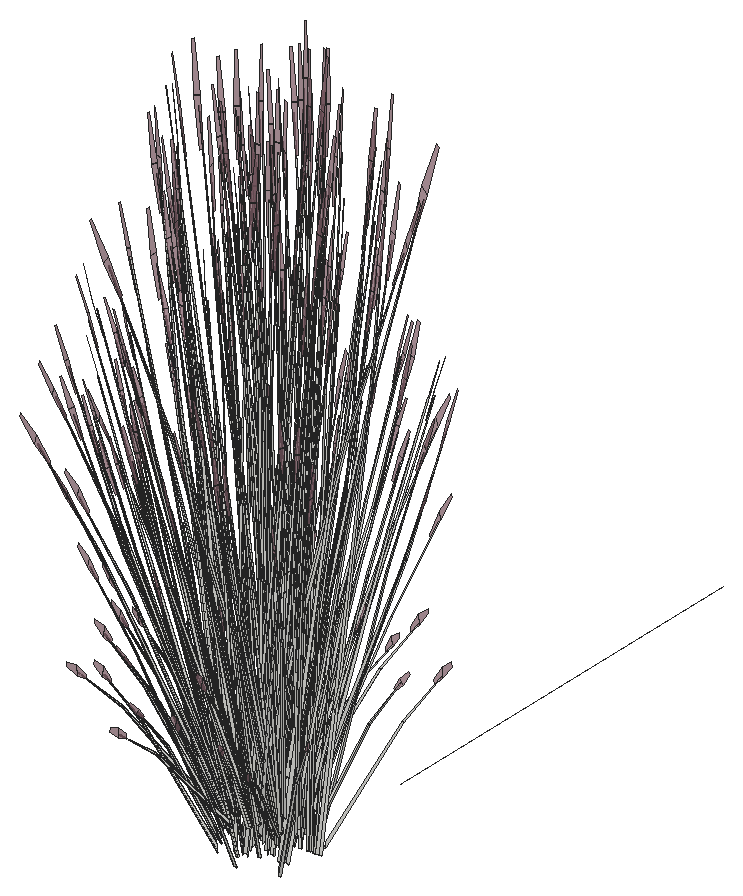
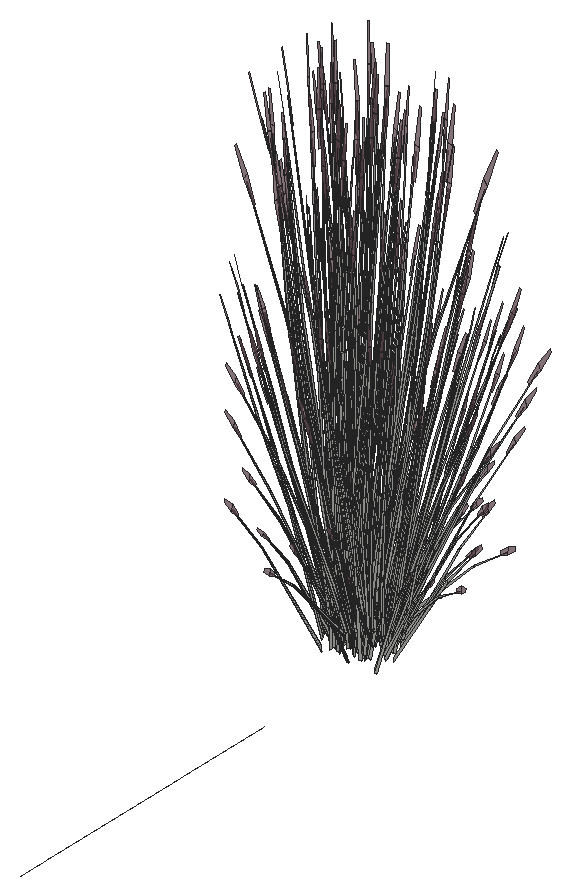
# SketchUp Ruby script. Lengths in inches.
U = 1.inch
M = Sketchup.active_model
def pt(a) = Geom::Point3d.new(a.map { |v| v * U })
def face(e, loops, mat)
  f = e.add_face(loops[0].map { |a| pt(a) })
  loops[1..].each { |l| e.add_face(l.map { |a| pt(a) }).erase! }
  f.material = f.back_material = mat if mat
  f
end
# faces: each face lists its corners as indices into pts; further lists are holes
def faces(e, pts, list, mat = nil) = list.each { |f| face(e, (f[0].is_a?(Array) ? f : [f]).map { |l| l.map { |i| pts[i] } }, mat) }
# xy, xz, yz: faces in a plane at the given z, y or x. An outline is a flat list of corners, or four numbers for a rectangle; further outlines are holes
def ring(l) = l.size == 4 ? [[l[0], l[1]], [l[2], l[1]], [l[2], l[3]], [l[0], l[3]]] : l.each_slice(2).to_a
def flat(e, list, mat, &to3) = list.each { |f| face(e, (f[0].is_a?(Array) ? f : [f]).map { |l| ring(l).map { |u, v| to3.(u, v) } }, mat) }
def xy(e, z, list, mat = nil) = flat(e, list, mat) { |x, y| [x, y, z] }
def xz(e, y, list, mat = nil) = flat(e, list, mat) { |x, z| [x, y, z] }
def yz(e, x, list, mat = nil) = flat(e, list, mat) { |y, z| [x, y, z] }
def lines(e, pts, list) = list.each { |a, b| e.add_line(pt(pts[a]), pt(pts[b])) }
# prism: a flat outline (further loops are holes) pulled along v
def prism(e, loops, v, mat = nil)
  f = face(e, loops, mat); d = Geom::Vector3d.new(v.map { |x| x * U })
  f.pushpull(f.normal.samedirection?(d) ? d.length : -d.length)
end
def box(e, o, s, mat = nil) = prism(e, [[o, [o[0] + s[0], o[1], o[2]], [o[0] + s[0], o[1] + s[1], o[2]], [o[0], o[1] + s[1], o[2]]]], [0, 0, s[2]], mat)
def at(x, y, z, deg = 0) = Geom::Transformation.translation(pt([x, y, z])) * Geom::Transformation.rotation(ORIGIN, Z_AXIS, deg.degrees)
def axes(o, x, y, z) = Geom::Transformation.new([*x, 0, *y, 0, *z, 0, *pt(o).to_a, 1])
def part(name) = M.definitions.add(name)
# library, detail: a bought-in or finely detailed component or shape, given as its bounding box
def library(name, o, s) = part(name).tap { |d| box(d.entities, o, s) }
def detail(e, o, s) = box(e.add_group.entities, o, s)
def put(e, d, t, mat = nil) = e.add_instance(d, t).tap { |i| i.material = mat if mat }
def group(e, t, mat = nil) = e.add_group.tap { |g| g.transformation = t; g.material = mat if mat }.entities
root = M.entities
M.materials.add("LightPink_Translucent").color = [144, 107, 117]
M.materials["LightPink_Translucent"].alpha = 0.75
c1 = part("blade")
p = [[2.15,0.21,22],[0,0.17,0],[0.09,0.45,0],[2.18,0.31,22],[2.29,0.31,22],[0.38,0.45,0],
  [2.48,0.24,33],[2.49,0.24,33],[2.48,0.22,33]]
faces(c1.entities,p,[[0,1,2,3],[4,5,2,3],[6,3,4,7],[8,0,3,6]])
c2 = part("seeds")
p = [[0.3,-0.1,1.38],[-0.01,-0.03,1.59],[-0.01,-0.03,0.03],[0.14,-0.07,-0.07],[0.29,-0.03,3],[0.15,0.01,3.11]]
faces(c2.entities,p,[[0,1,2,3],[1,0,4,5]],"LightPink_Translucent")
c3 = part("blade with seeds")
put(c3.entities,c1,at(0,0,0))
put(c3.entities,c2,axes([2.4,0.25,30.99],[1.5799,-0.05474,1.17369],[-0.12525,1.92788,0.29478],[-0.07173,-0.02425,1.56792]))
p = [[48,63.98,-6],[48,27.98,-6]]
lines(root,p,[[0,1]])
put(root,c3,axes([44.96,12.17,-2.125],[0.31515,-0.01384,1.71376],[-0.20907,0.5998,0.13857],[-0.44912,-0.0371,0.73262]))
put(root,c3,axes([45.09,13.23,-2.125],[0.26363,-0.12925,1.71376],[0.22195,0.59723,0.13857],[-0.41388,0.13498,0.73262]))
put(root,c3,axes([44.27,14.24,-3.41],[0.26405,0.05016,1.43002],[0.17019,0.51235,-0.30754],[-0.35868,0.0959,0.61141]))
put(root,c3,axes([46.61,12.6,-2.66],[0.21597,-0.08839,1.77064],[0.07448,0.61717,0.13857],[-0.4678,0.08189,0.63284]))
put(root,c3,axes([44.28,13.02,-1.28],[-0.12407,0.07933,1.74944],[0.01055,0.57963,-0.27667],[-0.2844,0.07538,0.14031]))
put(root,c3,axes([45.9,11.61,-1.02],[-0.75952,-0.01471,-0.71045],[0.05101,-0.61953,0.08574],[-0.32177,-0.06538,1.00501]))
put(root,c3,axes([45.29,11.76,-3.41],[0.14835,0.17012,1.43002],[-0.34183,0.46242,-0.30754],[-0.351,-0.11053,0.61141]))
put(root,c3,axes([44.68,12.6875,-1.47],[-0.63144,-0.17046,-0.35414],[0.18417,-0.49731,0.4572],[-0.25423,0.0456,0.87481]))
put(root,c3,axes([45.56,11.21,-2.125],[0.28223,0.10528,1.71376],[-0.58406,0.44165,0.13857],[-0.36402,-0.19924,0.73262]))
put(root,c3,axes([42.91,13.6,-1.29],[0.09697,0.01639,1.77383],[0.29997,0.53988,-0.16761],[-0.1985,0.1417,0.31391]))
put(root,c3,axes([45.12,12.94,-1.32],[-0.20584,0.55581,-0.51099],[-0.70573,-0.19051,-0.3958],[-0.28414,0.05097,0.97773]))
put(root,c3,axes([45.65,11.74,-1.32],[-0.55171,0.40476,-0.51099],[-0.48318,-0.42758,-0.3958],[-0.28031,-0.06159,0.97773]))
put(root,c3,axes([44.76,12.91,-4.51],[0.01927,0.0963,1.76342],[-0.38846,0.5029,-0.26939],[-0.27592,-0.02535,0.30037]))
put(root,c3,axes([44.87,10.6,-1.29],[0.05633,0.06098,1.77383],[-0.27155,0.54815,-0.16761],[-0.27501,0.00397,0.31391]))
put(root,c3,axes([43.72,15.32,-3.23],[0.31665,-0.27694,1.1486],[0.12495,0.43841,0.84392],[-0.22883,0.0785,0.25299]))
put(root,c3,axes([45.5,10.24,-1.28],[-0.16348,-0.00431,1.74944],[-0.52047,0.43131,-0.27667],[-0.2777,-0.08813,0.14031]))
put(root,c3,axes([44.83,12.625,-1.27],[0.21466,-0.55714,0.48003],[0.70573,0.19051,0.3958],[-0.27753,0.03348,0.9933]))
put(root,c3,axes([45.08,12.46,-0.97],[0.38229,0.5533,-0.1216],[-0.6785,0.2719,-0.67495],[-0.28593,0.073,1.02557]))
put(root,c3,axes([45.94,11.32,-0.97],[-0.04068,0.62141,-0.1216],[-0.77029,-0.01698,-0.67495],[-0.29667,-0.04317,1.02557]))
put(root,c3,axes([45.45,11.36,-1.47],[-0.43232,-0.38257,-0.35414],[0.49364,-0.36215,0.4572],[-0.25081,-0.0551,0.87481]))
put(root,c3,axes([44.78,12.48,-1.27],[-0.27906,-0.41663,0.0643],[0.50888,-0.20393,0.50621],[-0.22432,0.04024,0.77189]))
put(root,c3,axes([46.06,13.63,-2.125],[0.18977,-0.18775,1.71376],[0.47917,0.50677,0.13857],[-0.32866,0.23079,0.73262]))
put(root,c3,axes([44.91,14.12,-1.47],[-0.66138,0.08733,-0.35414],[-0.17464,-0.49921,0.4572],[-0.18953,0.13408,0.87481]))
put(root,c3,axes([44.55,15.6,-4.51],[0.10192,0.06105,1.76342],[0.17281,0.56562,-0.26939],[-0.22588,0.12062,0.30037]))
put(root,c3,axes([44.41,12.28,-3.23],[0.48508,-0.04372,1.1486],[-0.3077,0.38525,0.84392],[-0.23971,-0.05779,0.25299]))
put(root,c3,axes([45,14.01,-1.27],[-0.18844,-0.56237,0.48003],[0.73919,-0.0976,0.3958],[-0.21785,0.13226,0.9933]))
put(root,c3,axes([45.38,11.21,-0.91],[0.62747,-0.45094,0.53763],[0.54116,0.47889,0.4433],[-0.29439,-0.08318,1.11249]))
put(root,c3,axes([44.85,13.9,-1.27],[-0.52161,-0.25698,0.0643],[0.30368,-0.36595,0.50621],[-0.16723,0.11831,0.77189]))
put(root,c3,axes([45.91,14.09,-2.125],[0.14147,-0.21002,1.71376],[0.59349,0.43464,0.13857],[-0.26773,0.27089,0.73262]))
put(root,c3,axes([45.35,12.63,-0.95],[0.63144,0.17046,0.35414],[-0.18417,0.49731,-0.4572],[-0.25423,0.0456,0.87481]))
put(root,c3,axes([45.46,14.18,-1.32],[0.19519,0.55794,-0.51099],[-0.73919,0.0976,-0.3958],[-0.21183,0.14986,0.97773]))
put(root,c3,axes([45.67,11.21,-1.27],[0.03826,-0.46465,0.0643],[0.57772,0.01274,0.50621],[-0.2213,-0.04862,0.77189]))
put(root,c3,axes([44.31,15.18,-1.28],[-0.01889,0.12092,1.74944],[0.53598,0.42065,-0.27667],[-0.14032,0.19892,0.14031]))
put(root,c3,axes([47.3,13.78,-3.94],[-0.79037,-0.10018,-0.62353],[0.16679,-0.61794,-0.16365],[-0.23587,-0.07488,1.37633]))
put(root,c3,axes([47.44,10.41,-0.57],[-0.50709,0.58578,-0.13619],[-0.73436,-0.33748,-0.75594],[-0.25527,-0.1655,1.14864]))
put(root,c3,axes([46.06,11.56,-0.95],[0.43232,0.38257,0.35414],[-0.49364,0.36215,-0.4572],[-0.25081,-0.0551,0.87481]))
put(root,c3,axes([47.22,10.88,-1.02],[-0.64788,-0.29534,-0.71045],[0.46044,-0.51755,0.08574],[-0.23473,-0.17635,1.00501]))
put(root,c3,axes([46.92,10.9,-1.32],[-0.74975,0.14525,-0.51099],[-0.13115,-0.55007,-0.3958],[-0.20138,-0.15763,0.97773]))
put(root,c3,axes([46.27,14.95,-3.98],[-0.7111,-0.30552,-0.49651],[0.42504,-0.54784,0],[-0.16196,-0.06958,1.57504]))
put(root,c3,axes([45.95,10.4,-4.51],[-0.0736,0.08049,1.76342],[-0.74378,0.17355,-0.26939],[-0.17968,-0.15788,0.30037]))
put(root,c3,axes([45.11,13.78,-0.97],[0.70283,0.33692,-0.1216],[-0.40491,0.48793,-0.67495],[-0.19857,0.16961,1.02557]))
put(root,c3,axes([46.7,15.32,-3.625],[-0.47504,0.61229,0],[-0.79476,-0.34146,-0.51607],[-0.18101,-0.07777,1.63711]))
put(root,c3,axes([43.95,15.24,-0.35],[0.67048,0.16311,-0.06488],[-0.20625,0.50201,-0.29416],[-0.10966,0.07622,0.97024]))
put(root,c3,axes([45.45,13.83,-0.95],[0.66138,-0.08733,0.35414],[0.17464,0.49921,-0.4572],[-0.18953,0.13408,0.87481]))
put(root,c3,axes([45.83,16.2,-3.41],[0.23977,-0.09639,1.43002],[0.59198,0.29065,-0.30754],[-0.1762,0.25149,0.61141]))
put(root,c3,axes([45.49,10.71,-3.87],[-0.21918,0.49894,-0.03893],[-0.6746,-0.15348,-0.17649],[-0.10242,-0.08161,0.58215]))
put(root,c3,axes([47.25,9.02,-1.29],[-0.01417,0.07324,1.77383],[-0.6991,0.2658,-0.16761],[-0.20573,-0.13587,0.31391]))
put(root,c3,axes([46.5,10.08,-3.41],[-0.04601,0.19989,1.43002],[-0.67263,0.16733,-0.30754],[-0.15723,-0.25836,0.61141]))
put(root,c3,axes([46.72,10.6,-2.125],[0.17368,0.19618,1.71376],[-0.80256,0.16516,0.13857],[-0.18139,-0.30799,0.73262]))
put(root,c3,axes([48.2,13.87,-3.33],[-0.76714,0.40567,-0.29095],[-0.51013,-0.57321,-0.50002],[-0.18927,-0.05821,1.59708]))
put(root,c3,axes([46.08,15.15,-1.27],[-0.54105,-0.41691,0.48003],[0.57458,-0.35956,0.3958],[-0.0998,0.1956,0.9933]))
put(root,c3,axes([47,10.49,-1.47],[-0.11735,-0.49217,-0.35414],[0.67083,-0.12996,0.4572],[-0.18018,-0.14104,0.87481]))
put(root,c3,axes([45.13,12.99,-3.625],[-0.95008,0,0],[0,-0.68292,-0.51607],[0,-0.15554,1.63711]))
put(root,c3,axes([46.46,14.72,-3.97],[-0.17848,-0.53243,-0.30978],[0.70886,-0.15119,0.30978],[-0.1429,-0.0614,1.38974]))
put(root,c3,axes([45.88,15.11,-1.27],[-0.62439,-0.02847,0.0643],[0.01712,-0.42991,0.50621],[-0.06534,0.16468,0.77189]))
put(root,c3,axes([46.08,15.28,-1.47],[-0.5141,0.32171,-0.35414],[-0.48666,-0.36734,0.4572],[-0.07405,0.18664,0.87481]))
put(root,c3,axes([48.71,14.3125,-3.94],[-0.51177,0.45928,-0.62353],[-0.63575,-0.41646,-0.16365],[-0.20507,0.11457,1.37633]))
put(root,c3,axes([47.4,10.89,-0.95],[0.11735,0.49217,0.35414],[-0.67083,0.12996,-0.4572],[-0.18018,-0.14104,0.87481]))
put(root,c3,axes([44.24,16.42,-1.29],[0.0862,-0.03689,1.77383],[0.71245,0.24539,-0.16761],[-0.01674,0.20431,0.31391]))
put(root,c3,axes([45.86,12.81,-3.67],[-0.70674,0.51372,0.30756],[-0.70717,-0.50832,-0.36492],[-0.02468,-0.14589,1.64885]))
put(root,c3,axes([48.77,14.22,-2.67],[0.65659,0.2464,1.51261],[-0.64324,0.53082,0.59816],[-0.28812,-0.31461,1.26806]))
put(root,c3,axes([46.27,9.76,-3.23],[0.39634,0.21267,1.1486],[-0.57721,0.12784,0.84392],[-0.1235,-0.16344,0.25299]))
put(root,c3,axes([49.0625,14.05,-3.54],[-0.74193,-0.49181,-0.25192],[0.6243,-0.55226,0.5513],[-0.19979,0.05753,1.68216]))
put(root,c3,axes([47.71,13.58,-3.79],[-0.45644,-0.51287,-0.44739],[0.69137,-0.36116,0.21531],[-0.14771,-0.06346,1.43643]))
put(root,c3,axes([46.42,14.9375,-0.66],[-0.01977,0.56521,-0.7886],[-0.83252,-0.03796,0.09517],[-0.08786,0.23945,1.11556]))
put(root,c3,axes([46.41,16.53,-3.23],[-0.01966,-0.36332,1.1486],[0.49135,0.25914,0.84392],[-0.09663,0.17317,0.25299]))
put(root,c3,axes([47.09,10.31,-0.91],[0.84639,-0.15705,0.53763],[0.14689,0.61608,0.4433],[-0.19906,-0.18157,1.11249]))
put(root,c3,axes([48.68,13.95,-3.79],[-0.82508,0.03772,-0.44739],[-0.07462,-0.62614,0.21531],[-0.14771,0.06346,1.43643]))
put(root,c3,axes([47.29,10.45,-1.27],[0.34533,-0.38816,0.0643],[0.49176,0.22599,0.50621],[-0.15898,-0.12445,0.77189]))
put(root,c3,axes([47.11,15,-3.52],[0.7111,0.30552,0.49651],[-0.42504,0.54784,0],[-0.16196,-0.06958,1.57504]))
put(root,c3,axes([46.14,15.73,-2.64],[0.01669,-0.31544,1.54345],[0.75083,0.16661,0.21329],[-0.06506,0.33618,0.72882]))
put(root,c3,axes([47.78,13.875,-3.5625],[0.20138,-0.72405,-0.23429],[0.95485,0.12621,0.51271],[-0.16685,-0.09999,1.5644]))
put(root,c3,axes([48.125,14.05,-3.38],[-0.14658,0.54532,0.1448],[-0.71613,-0.09466,-0.41347],[-0.13033,-0.05599,1.26744]))
put(root,c3,axes([48.04,9.3,-1.28],[-0.11621,-0.08567,1.74944],[-0.77555,0.05431,-0.27667],[-0.12378,-0.20491,0.14031]))
put(root,c3,axes([49.55,15.57,-3.98],[-0.7111,0.30552,-0.49651],[-0.42504,-0.54784,0],[-0.16196,0.06958,1.57504]))
put(root,c3,axes([45.34,12.52,-3.98],[0,-0.61104,-0.49651],[0.85008,0,0],[0,-0.13917,1.57504]))
put(root,c3,axes([45.71,13.09,-3.52],[0,0.61104,0.49651],[-0.85008,0,0],[0,-0.13917,1.57504]))
put(root,c3,axes([49.6,15.4,-3.81],[-0.46912,-0.61443,-0.05142],[0.79476,-0.34146,0.51607],[-0.19584,0.0585,1.6363]))
put(root,c3,axes([46.59,15.125,-1],[0.54391,0.41056,-0.5672],[-0.57458,0.35956,-0.43934],[-0.08276,0.2086,1.08528]))
put(root,c3,axes([49.38,15.32,-3.97],[-0.70886,-0.15119,-0.30978],[0.17848,-0.53243,0.30978],[-0.1429,0.0614,1.38974]))
put(root,c3,axes([46.35,14.82,-0.95],[0.5141,-0.32171,0.35414],[0.48666,0.36734,-0.4572],[-0.07405,0.18664,0.87481]))
put(root,c3,axes([47.5625,13.23,-3.33],[-0.85568,-0.29155,-0.29095],[0.41201,-0.61537,-0.50002],[-0.02689,-0.15109,1.59708]))
put(root,c3,axes([49.79,13.05,-3.16],[-0.02076,-0.57531,1.41272],[0.93937,0.14913,0.59816],[-0.22217,0.31481,1.3335]))
put(root,c3,axes([46.02,14.91,-0.6],[0.83505,0.03027,-0.13498],[-0.02282,0.57322,-0.74919],[-0.05801,0.22077,1.13838]))
put(root,c3,axes([46,15.74,-3.18],[0.69024,-0.1082,0.06507],[0.15868,0.43593,-0.86304],[-0.04376,0.22067,0.7736]))
put(root,c3,axes([49.26,13.78,-3.33],[0.08854,0.69723,-0.29095],[-0.92215,0.04216,-0.50002],[-0.16238,0.09287,1.59708]))
put(root,c3,axes([47.18,12.61,-3.9],[-0.31203,-0.62659,-0.69835],[0.89884,-0.22566,-0.18329],[-0.03449,-0.21218,1.54149]))
put(root,c3,axes([49.22,10.62,-0.97],[-0.74352,0.28449,-0.1216],[-0.36538,-0.50492,-0.67495],[-0.0981,-0.21277,1.02557]))
put(root,c3,axes([48.59,10.64,-1.32],[-0.7469,-0.15318,-0.51099],[0.25601,-0.52518,-0.3958],[-0.06849,-0.21144,0.97773]))
put(root,c3,axes([47.21,14.54,-2.125],[-0.0186,-0.23452,1.71376],[0.80601,0.15558,0.13857],[-0.04985,0.33422,0.73262]))
put(root,c3,axes([45.71,12.54,-3.97],[0.53038,-0.38124,-0.30978],[0.53038,0.38124,0.30978],[0,-0.1228,1.38974]))
put(root,c3,axes([48.1,10.07,-3.87],[-0.52505,0.35054,-0.03893],[-0.48109,-0.38392,-0.17649],[-0.03387,-0.10878,0.58215]))
put(root,c3,axes([47.89,13.53,-3.64],[0.96033,0.12874,0.45755],[-0.19544,0.7271,0.17955],[-0.14034,-0.07021,1.58856]))
put(root,c3,axes([47.64,13.4,-3.28],[-0.36864,0.55059,0.44739],[-0.76598,-0.26498,-0.21531],[0,-0.12692,1.43643]))
put(root,c3,axes([48.86,10.74,-1.02],[-0.36264,-0.49684,-0.71045],[0.74649,-0.27689,0.08574],[-0.0848,-0.24006,1.00501]))
put(root,c3,axes([47.375,14.6875,-3.53],[0.81646,-0.16218,0.17642],[0.20161,0.60355,0.35086],[-0.07282,-0.08794,1.60407]))
put(root,c3,axes([48.42,14.78,-3.8],[-0.76598,-0.27433,0],[0.36864,-0.57001,0],[0,0,1.62707]))
put(root,c3,axes([49,10.82,-0.95],[-0.22906,0.4699,0.35414],[-0.66828,-0.13705,-0.4572],[-0.06128,-0.18919,0.87481]))
put(root,c3,axes([50.2,15.47,-3.625],[0.47504,0.61229,0],[-0.79476,0.34146,-0.51607],[-0.18101,0.07777,1.63711]))
put(root,c3,axes([47.78,15.73,-0.9375],[-0.74868,-0.15974,0.53283],[0.25601,-0.52518,0.43934],[0.04499,0.20653,1.10256]))
put(root,c3,axes([47.58,15.77,-1.27],[-0.55987,0.20767,0.0643],[-0.27403,-0.37869,0.50621],[0.05407,0.16693,0.77189]))
put(root,c3,axes([49.8,14.72,-3.53],[0.21949,-0.60727,0.17642],[0.8032,0.17185,0.35086],[-0.13875,0.00296,1.60407]))
put(root,c3,axes([49.43,13.92,-3.38],[0.56134,0.36712,0.1448],[-0.46823,0.41419,-0.41347],[-0.13033,0.05599,1.26744]))
put(root,c3,axes([49.23,13.46,-3.7],[-0.70674,-0.52593,-0.06131],[0.70717,-0.52625,0],[-0.02468,-0.01837,1.75571]))
put(root,c3,axes([49.42,13.65,-3.28],[0.82508,-0.03772,0.44739],[0.07462,0.62614,-0.21531],[-0.14771,0.06346,1.43643]))
put(root,c3,axes([49.62,15.09,-3.67],[0.95122,0.19861,0.30756],[-0.23797,0.7099,-0.36492],[-0.15744,0.08885,1.64885]))
put(root,c3,axes([48.23,9.64,-4.51],[-0.12744,0.02202,1.76342],[-0.70477,-0.24781,-0.26939],[0.01183,-0.2067,0.30037]))
put(root,c3,axes([50.03,15.05,-3.52],[0.7111,-0.30552,0.49651],[0.42504,0.54784,0],[-0.16196,0.06958,1.57504]))
put(root,c3,axes([48.93,10.32,-1.47],[0.22906,-0.4699,-0.35414],[0.66828,0.13705,0.4572],[-0.06128,-0.18919,0.87481]))
put(root,c3,axes([47.81,12.86,-3.64],[0.33034,0.68327,0.45755],[-0.94388,0.2376,0.17955],[0.01154,-0.12555,1.58856]))
put(root,c3,axes([47.66,12.77,-3.79],[0.36864,-0.55059,-0.44739],[0.76598,0.26498,0.21531],[0,-0.12692,1.43643]))
put(root,c3,axes([48.6,14.55,-3.8],[-0.24791,-0.5268,0],[0.70791,-0.18448,0],[0,0,1.54371]))
put(root,c3,axes([47.7,15.66,-4.51],[0.12297,-0.03325,1.76342],[0.73967,0.18301,-0.26939],[0.02163,0.20626,0.30037]))
put(root,c3,axes([47.86,15.84,-1.47],[-0.22906,0.4699,-0.35414],[-0.66828,-0.13705,0.4572],[0.06128,0.18919,0.87481]))
put(root,c3,axes([49.6,13.51,-3.79],[-0.36864,0.55059,-0.44739],[-0.76598,-0.26498,0.21531],[0,0.12692,1.43643]))
put(root,c3,axes([49.21,10.39,-1.27],[0.55987,-0.20767,0.0643],[0.27403,0.37869,0.50621],[-0.05407,-0.16693,0.77189]))
put(root,c3,axes([47.39,16.68,-1.28],[0.09631,0.0984,1.74944],[0.77725,0.03866,-0.27667],[0.07816,0.217,0.14031]))
put(root,c3,axes([51.06,13.17,-3.53],[-0.59697,-0.44509,0.17642],[0.60159,-0.4317,0.35086],[-0.06593,0.0909,1.60407]))
put(root,c3,axes([49,12.92,-3.79],[0,-0.70701,0],[0.95008,0,0],[0,0,1.79456]))
put(root,c3,axes([49.01,10.43,-1.27],[0.74868,0.15974,0.48003],[-0.25601,0.52518,0.3958],[-0.04499,-0.20653,0.9933]))
put(root,c3,axes([48.11,13.04,-3.57],[0.8561,0.29616,0.24065],[-0.41201,0.61537,0.50002],[0,-0.14185,1.60543]))
put(root,c3,axes([49.47,13.2,-3.71],[0,0.70667,-0.05637],[-0.95008,0,0],[0,0.02221,1.79368]))
put(root,c3,axes([47.84,12.63,-3.28],[-0.82508,0.03772,0.44739],[-0.07462,-0.62614,-0.21531],[0.14771,-0.06346,1.43643]))
put(root,c3,axes([47.79,15.35,-0.95],[0.22906,-0.4699,0.35414],[0.66828,0.13705,-0.4572],[0.06128,0.18919,0.87481]))
put(root,c3,axes([47.45,11.56,-3.53],[-0.21949,0.60727,0.17642],[-0.8032,-0.17185,0.35086],[0.13875,-0.00296,1.60407]))
put(root,c3,axes([49.02,14.57,-3.71],[0.33034,0.70197,-0.06012],[-0.94388,0.24598,0],[0.01154,0.02451,1.72173]))
put(root,c3,axes([47.06,10.81,-3.625],[-0.47504,-0.61229,0],[0.79476,-0.34146,-0.51607],[0.18101,-0.07777,1.63711]))
put(root,c3,axes([47.93,15.42,-1.02],[0.36264,0.49684,-0.71045],[-0.74649,0.27689,0.08574],[0.0848,0.24006,1.00501]))
put(root,c3,axes([51.75,13.64,-3.8],[-0.94962,-0.00489,-0.04976],[0,-0.68292,0.49943],[-0.02984,0.15546,1.58352]))
put(root,c3,axes([49.88,11.59,-3.53],[-0.81646,0.16218,0.17642],[-0.20161,-0.60355,0.35086],[0.07282,0.08794,1.60407]))
put(root,c3,axes([49.05,9.33,-3.23],[0.09747,0.35631,1.1486],[-0.54071,-0.19735,0.84392],[0.05818,-0.18244,0.25299]))
put(root,c3,axes([48.6875,17.03,-0.35],[0.52505,-0.35054,-0.06488],[0.48109,0.38392,-0.29416],[0.03387,0.10878,0.97024]))
put(root,c3,axes([48.54,12.47,-3.64],[-0.62999,0.55453,0.45755],[-0.74845,-0.4895,0.17955],[0.15188,-0.05534,1.58856]))
put(root,c3,axes([49.62,13.34,-3.79],[0.53038,0.39469,0],[-0.53038,0.39469,0],[0,0,1.69266]))
put(root,c3,axes([49.61,12.88,-3.28],[0.36864,-0.55059,0.44739],[0.76598,0.26498,-0.21531],[0,0.12692,1.43643]))
put(root,c3,axes([49.29,14.8,-3.8],[0.76598,0.27433,0],[-0.36864,0.57001,0],[0,0,1.74954]))
put(root,c3,axes([48.2,15.52,-1.32],[0.7469,0.15318,-0.51099],[-0.25601,0.52518,-0.3958],[0.06849,0.21144,0.97773]))
put(root,c3,axes([47.5625,15.55,-0.97],[0.74352,-0.28449,-0.1216],[0.36538,0.50492,-0.67495],[0.0981,0.21277,1.02557]))
put(root,c3,axes([49.37,12.75,-3.62],[-0.96033,-0.12874,0.49198],[0.19544,-0.7271,0.19306],[0.14034,0.07021,1.70813]))
put(root,c3,axes([51.36,9.91,-1.29],[-0.07716,0.04667,1.77383],[-0.75601,-0.15746,-0.16761],[-0.02737,-0.20368,0.31391]))
put(root,c3,axes([50.77,11.26,-0.97],[-0.83505,-0.03027,-0.1216],[0.02282,-0.57322,-0.67495],[0.05801,-0.22077,1.02557]))
put(root,c3,axes([51.55,13.74,-3.97],[-0.53038,0.38124,-0.30978],[-0.53038,-0.38124,0.30978],[0,0.1228,1.38974]))
put(root,c3,axes([50.03,13.67,-3.91],[0.2786,0.55945,-0.69212],[-0.80253,0.20149,-0.18165],[0.03079,0.18945,1.52773]))
put(root,c3,axes([49.64,13.07,-3.79],[0.85008,0,0],[0,0.63259,0],[0,0,1.78407]))
put(root,c3,axes([50.44,11.35,-0.95],[-0.5141,0.32171,0.35414],[-0.48666,-0.36734,-0.4572],[0.07405,-0.18664,0.87481]))
put(root,c3,axes([48.82,12.375,-3.28],[-0.45644,-0.51287,0.44739],[0.69137,-0.36116,-0.21531],[0.14771,0.06346,1.43643]))
put(root,c3,axes([47.99,12.5,-3.33],[-0.08854,-0.69723,-0.29095],[0.92215,-0.04216,-0.50002],[0.16238,-0.09287,1.59708]))
put(root,c3,axes([49.93,13.01,-3.38],[0.70791,-0.1782,0.1448],[0.24791,0.50885,-0.41347],[0,0.11199,1.26744]))
put(root,c3,axes([50.2,11.04,-1.32],[-0.54391,-0.41056,-0.51099],[0.57458,-0.35956,-0.3958],[0.08276,-0.2086,0.97773]))
put(root,c3,axes([49.69,13.05,-3.33],[0.85568,0.29155,-0.29095],[-0.41201,0.61537,-0.50002],[0.02689,0.15109,1.59708]))
put(root,c3,axes([47.87,10.95,-3.97],[0.70886,0.15119,-0.30978],[-0.17848,0.53243,0.30978],[0.1429,-0.0614,1.38974]))
put(root,c3,axes([49.84,10.3125,-3.41],[-0.21597,0.12368,1.43002],[-0.64681,-0.21647,-0.30754],[0.1199,-0.26922,0.61141]))
put(root,c3,axes([51.55,13.19,-3.52],[0,-0.61104,0.49651],[0.85008,0,0],[0,0.13917,1.57504]))
put(root,c3,axes([51.91,13.76,-3.98],[0,0.61104,-0.49651],[-0.85008,0,0],[0,0.13917,1.57504]))
put(root,c3,axes([49.64,15.61,-1.27],[-0.75571,0.14023,0.48003],[-0.13115,-0.55007,0.3958],[0.17773,0.16212,0.9933]))
put(root,c3,axes([47.7,10.71,-3.98],[0.7111,-0.30552,-0.49651],[0.42504,0.54784,0],[0.16196,-0.06958,1.57504]))
put(root,c3,axes([49.5,15.72,-1.27],[-0.34533,0.38816,0.0643],[-0.49176,-0.22599,0.50621],[0.15898,0.12445,0.77189]))
put(root,c3,axes([48.625,14.4375,-2.125],[-0.17368,-0.19618,1.71376],[0.80256,-0.16516,0.13857],[0.18139,0.30799,0.73262]))
put(root,c3,axes([49.13,12.23,-3.38],[0.14658,-0.54532,0.1448],[0.71613,0.09466,-0.41347],[0.13033,0.05599,1.26744]))
put(root,c3,axes([50.15,11.28,-3.52],[-0.7111,-0.30552,0.49651],[0.42504,-0.54784,0],[0.16196,0.06958,1.57504]))
put(root,c3,axes([50.37,11.23,-1.02],[0.01977,-0.56521,-0.71045],[0.83252,0.03796,0.08574],[0.08786,-0.23945,1.00501]))
put(root,c3,axes([49.53,14.47,-3.82],[0.79769,-0.20732,-0.19198],[0.2803,0.59721,0.00008],[0.08805,-0.02292,1.73897]))
put(root,c3,axes([49.39,15.27,-0.95],[-0.11735,-0.49217,0.35414],[0.67083,-0.12996,-0.4572],[0.18018,0.14104,0.87481]))
put(root,c3,axes([49.54,12.7,-3.79],[0.45644,0.51287,-0.44739],[-0.69137,0.36116,0.21531],[0.14771,0.06346,1.43643]))
put(root,c3,axes([49.84,12.44,-1.53],[-0.65655,-0.31748,1.38283],[0.69326,-0.49431,0.59665],[0.21183,0.29789,1.33663]))
put(root,c3,axes([50.71,10.89,-1.47],[0.5141,-0.32171,-0.35414],[0.48666,0.36734,0.4572],[0.07405,-0.18664,0.87481]))
put(root,c3,axes([48.74,15.96,-1.29],[0.00225,-0.07398,1.77383],[0.65113,-0.32638,-0.16761],[0.22617,0.1165,0.31391]))
put(root,c3,axes([50.91,11.05,-1.27],[0.62439,0.02847,0.0643],[-0.01712,0.42991,0.50621],[0.06534,-0.16468,0.77189]))
put(root,c3,axes([50.83,15.02,-3.23],[-0.4278,-0.1757,1.1486],[0.5524,-0.17852,0.84392],[0.14899,0.15122,0.25299]))
put(root,c3,axes([49.3125,14.84,-3.41],[0.01341,-0.20255,1.43002],[0.64074,-0.22625,-0.30754],[0.1978,0.24243,0.61141]))
put(root,c3,axes([51.53,10.35,-1.28],[-0.00733,-0.12161,1.74944],[-0.61946,-0.35147,-0.27667],[0.09577,-0.21306,0.14031]))
put(root,c3,axes([48.55,11.97,-3.94],[0.51177,-0.45928,-0.62353],[0.63575,0.41646,-0.16365],[0.20507,-0.11457,1.37633]))
put(root,c3,axes([50.71,11.01,-1.27],[0.54105,0.41691,0.48003],[-0.57458,0.35956,0.3958],[0.0998,-0.1956,0.9933]))
put(root,c3,axes([50.79,11.56,-3.97],[0.17848,0.53243,-0.30978],[-0.70886,0.15119,0.30978],[0.1429,0.0614,1.38974]))
put(root,c3,axes([52.125,13.29,-3.625],[0.95008,0,0],[0,0.68292,-0.51607],[0,0.15554,1.63711]))
put(root,c3,axes([49.06,12.41,-3.33],[0.76714,-0.40567,-0.29095],[0.51013,0.57321,-0.50002],[0.18927,0.05821,1.59708]))
put(root,c3,axes([50.9,15.82,-3.33],[-0.48723,-0.01916,1.0506],[0.32177,-0.40701,0.58006],[0.19248,0.1446,0.8241]))
put(root,c3,axes([51.33,12.34,-0.95],[-0.66138,0.08733,0.35414],[-0.17464,-0.49921,-0.4572],[0.18953,-0.13408,0.87481]))
put(root,c3,axes([49.43,10.94,-2.125],[-0.14147,0.21002,1.71376],[-0.59349,-0.43464,0.13857],[0.26773,-0.27089,0.73262]))
put(root,c3,axes([49.33,15.53,-0.97],[0.45276,-0.52302,-0.1216],[0.65568,0.30132,-0.67495],[0.22792,0.14777,1.02557]))
put(root,c3,axes([47.12,12.05,-4.41],[-0.74787,0.24464,1.28929],[-0.23804,-0.70192,0.50096],[0.45924,0.01168,1.46642]))
put(root,c3,axes([51.68,12.39,-0.97],[-0.70283,-0.33692,-0.1216],[0.40491,-0.48793,-0.67495],[0.19857,-0.16961,1.02557]))
put(root,c3,axes([49.87,15.27,-1.32],[0.74975,-0.14525,-0.51099],[0.13115,0.55007,-0.3958],[0.20138,0.15763,0.97773]))
put(root,c3,axes([50.56,10.96,-3.625],[0.47504,-0.61229,0],[0.79476,0.34146,-0.51607],[0.18101,0.07777,1.63711]))
put(root,c3,axes([51.35,10.69,-4.51],[-0.11372,-0.04814,1.76342],[-0.29211,-0.53779,-0.26939],[0.19706,-0.14594,0.30037]))
put(root,c3,axes([50.73,14.61,-0.95],[-0.43232,-0.38257,0.35414],[0.49364,-0.36215,-0.4572],[0.25081,0.0551,0.87481]))
put(root,c3,axes([50.99,11.33,-3.98],[0.7111,0.30552,-0.49651],[-0.42504,0.54784,0],[0.16196,0.06958,1.57504]))
put(root,c3,axes([51.12,14.95,-1.27],[-0.03826,0.46465,0.0643],[-0.57772,-0.01274,0.50621],[0.2213,0.04862,0.77189]))
put(root,c3,axes([50.95,15.68,-4.51],[0.05536,-0.08822,1.76342],[0.69692,-0.25981,-0.26939],[0.21129,0.13447,0.30037]))
put(root,c3,axes([51.17,14.81,-1.27],[-0.56024,0.40262,0.48003],[-0.48318,-0.42758,0.3958],[0.26285,0.07427,0.9933]))
put(root,c3,axes([51.33,11.99,-1.32],[-0.19519,-0.55794,-0.51099],[0.73919,-0.0976,-0.3958],[0.21183,-0.14986,0.97773]))
